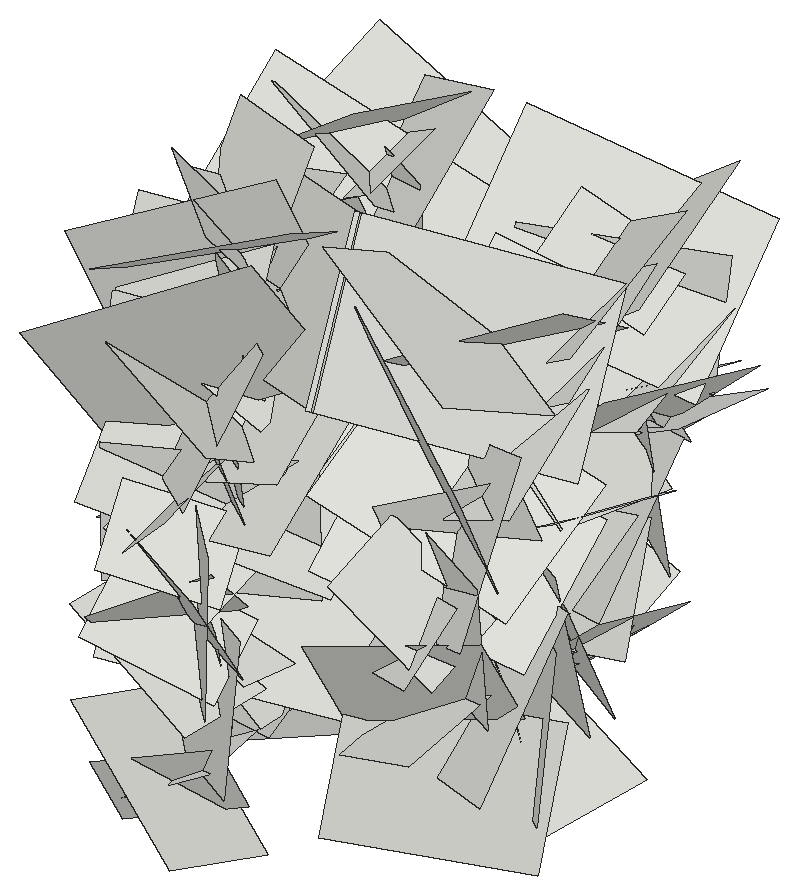
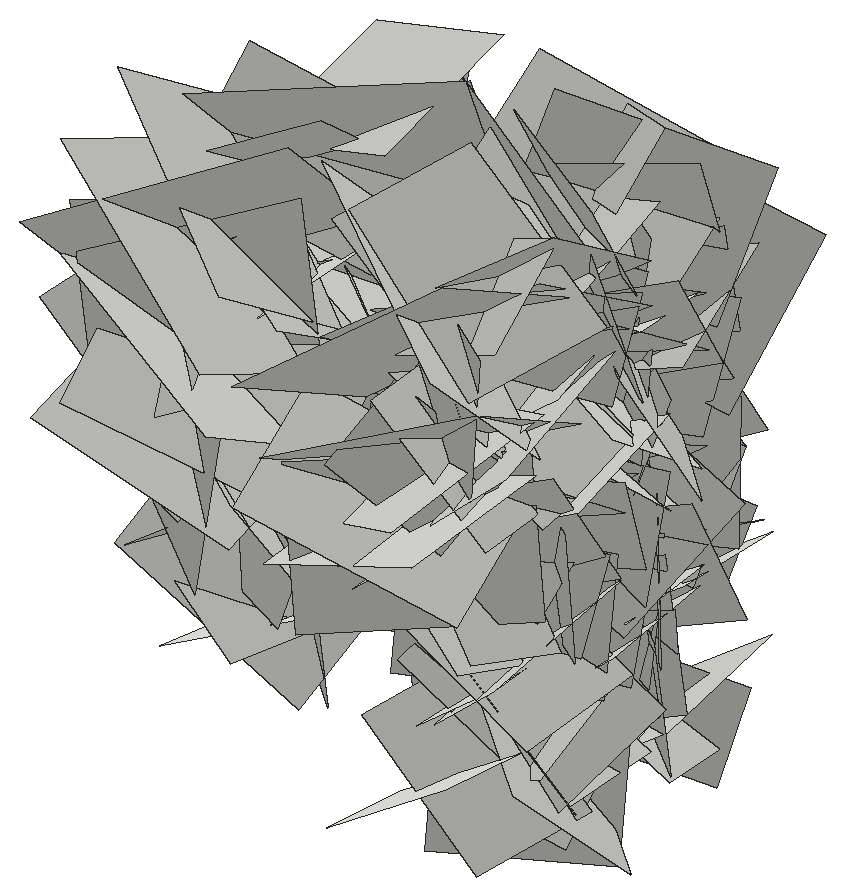
# SketchUp Ruby script. Lengths in inches.
U = 1.inch
M = Sketchup.active_model
def pt(a) = Geom::Point3d.new(a.map { |v| v * U })
def face(e, loops, mat)
  f = e.add_face(loops[0].map { |a| pt(a) })
  loops[1..].each { |l| e.add_face(l.map { |a| pt(a) }).erase! }
  f.material = f.back_material = mat if mat
  f
end
# faces: each face lists its corners as indices into pts; further lists are holes
def faces(e, pts, list, mat = nil) = list.each { |f| face(e, (f[0].is_a?(Array) ? f : [f]).map { |l| l.map { |i| pts[i] } }, mat) }
# xy, xz, yz: faces in a plane at the given z, y or x. An outline is a flat list of corners, or four numbers for a rectangle; further outlines are holes
def ring(l) = l.size == 4 ? [[l[0], l[1]], [l[2], l[1]], [l[2], l[3]], [l[0], l[3]]] : l.each_slice(2).to_a
def flat(e, list, mat, &to3) = list.each { |f| face(e, (f[0].is_a?(Array) ? f : [f]).map { |l| ring(l).map { |u, v| to3.(u, v) } }, mat) }
def xy(e, z, list, mat = nil) = flat(e, list, mat) { |x, y| [x, y, z] }
def xz(e, y, list, mat = nil) = flat(e, list, mat) { |x, z| [x, y, z] }
def yz(e, x, list, mat = nil) = flat(e, list, mat) { |y, z| [x, y, z] }
def lines(e, pts, list) = list.each { |a, b| e.add_line(pt(pts[a]), pt(pts[b])) }
# prism: a flat outline (further loops are holes) pulled along v
def prism(e, loops, v, mat = nil)
  f = face(e, loops, mat); d = Geom::Vector3d.new(v.map { |x| x * U })
  f.pushpull(f.normal.samedirection?(d) ? d.length : -d.length)
end
def box(e, o, s, mat = nil) = prism(e, [[o, [o[0] + s[0], o[1], o[2]], [o[0] + s[0], o[1] + s[1], o[2]], [o[0], o[1] + s[1], o[2]]]], [0, 0, s[2]], mat)
def at(x, y, z, deg = 0) = Geom::Transformation.translation(pt([x, y, z])) * Geom::Transformation.rotation(ORIGIN, Z_AXIS, deg.degrees)
def axes(o, x, y, z) = Geom::Transformation.new([*x, 0, *y, 0, *z, 0, *pt(o).to_a, 1])
def part(name) = M.definitions.add(name)
# library, detail: a bought-in or finely detailed component or shape, given as its bounding box
def library(name, o, s) = part(name).tap { |d| box(d.entities, o, s) }
def detail(e, o, s) = box(e.add_group.entities, o, s)
def put(e, d, t, mat = nil) = e.add_instance(d, t).tap { |i| i.material = mat if mat }
def group(e, t, mat = nil) = e.add_group.tap { |g| g.transformation = t; g.material = mat if mat }.entities
root = M.entities
c1 = part("Component\#6")
p = [[0.01,0,0],[0,3.24,4.54],[4.32,3.24,4.54],[4.33,0,0]]
faces(c1.entities,p,[[0,1,2,3]])
put(root,c1,axes([414.68,184.92,37.05],[-0.01613,-0.13323,-0.78421],[-0.01491,-0.78419,0.1335],[-0.84304,0.01642,0.01265]))
put(root,c1,axes([414.68,184.52,38.07],[0.06477,0.36641,0.7198],[-0.11209,0.71927,-0.35717],[-0.84878,-0.06703,0.10209]))
put(root,c1,axes([414.68,187.74,23.43],[0.08523,-0.9506,0.05636],[0.09187,0.06363,0.94959],[-1.00521,-0.07479,0.09156]))
put(root,c1,axes([410.71,187.08,35.11],[-0.23629,-0.52338,-1.02054],[-0.13084,-1.02265,0.55142],[1.20867,-0.21302,-0.13982]))
put(root,c1,axes([414.68,188.23,41.22],[0.26749,1.02168,-0.17372],[-0.00845,-0.17688,-1.05183],[-1.0985,0.25014,-0.03421]))
put(root,c1,axes([410.71,185.86,28.71],[-0.06844,0.29244,0.76285],[0.17475,0.75415,-0.27515],[0.84819,-0.13178,0.11824]))
put(root,c1,axes([410.71,192.58,32.17],[0.11188,-0.86522,-0.03173],[-0.14554,-0.04829,0.85998],[0.90613,0.09907,0.14204]))
put(root,c1,axes([410.71,189.53,40.3125],[-0.07096,0.70634,-0.4758],[0.12627,-0.46481,-0.70678],[0.89387,0.12173,0.06207]))
put(root,c1,axes([410.71,180.54,27.52],[0.00647,0.86334,-0.00303],[-0.00368,-0.003,-0.86336],[0.91514,-0.00612,-0.00345]))
put(root,c1,axes([414.68,184.84,39.1],[-0.02023,-0.20369,-0.6632],[-0.11732,-0.65406,0.20407],[-0.72599,0.11137,-0.0145]))
put(root,c1,axes([414.68,187.61,26.86],[0.07932,-0.16974,-0.83453],[0.0041,-0.83766,0.17072],[-0.9027,-0.01872,-0.07255]))
put(root,c1,axes([414.68,187.84,31.26],[-0.01205,0.8882,0.30464],[0.22592,0.29915,-0.86424],[-0.96935,0.05868,-0.20521]))
put(root,c1,axes([410.71,187.32,34.27],[0.05201,-0.4187,0.7383],[-0.02779,0.73844,0.42051],[0.89926,0.04704,-0.0297]))
put(root,c1,axes([414.68,182.78,23.92],[0.06221,-0.24398,0.83625],[0.07047,0.83695,0.23952],[-0.92069,0.04758,0.07484]))
put(root,c1,axes([410.71,186.99,20.26],[0.04681,-0.17583,0.86867],[-0.05724,0.86759,0.17835],[0.93771,0.06173,-0.03248]))
put(root,c1,axes([414.68,186.98,23.44],[0.07046,0.41434,0.63319],[-0.10971,0.63463,-0.40442],[-0.79457,-0.05088,0.11199]))
put(root,c1,axes([410.71,189.58,22.99],[-0.08755,-0.94666,0.34405],[-0.04779,0.34833,0.94763],[1.06661,-0.0621,0.0707]))
put(root,c1,axes([414.68,194.3125,23.26],[0.02367,-0.75059,-0.08188],[-0.02978,-0.08269,0.75031],[-0.79979,-0.01914,-0.03036]))
put(root,c1,axes([410.71,191.48,24.4],[-0.24044,-0.84726,-0.84182],[-0.11443,-0.83882,0.87332],[1.26085,-0.2377,-0.08127]))
put(root,c1,axes([410.71,182.91,34.72],[-0.14912,-0.41506,0.98502],[-0.044,0.99488,0.41329],[1.13217,-0.016,0.1458]))
put(root,c1,axes([414.68,183.3,35.54],[-0.06853,-0.0517,0.64839],[-0.02911,0.65122,0.04919],[-0.68886,-0.02238,-0.06659]))
put(root,c1,axes([414.68,186.9,33.68],[0.12726,-0.80704,-0.07778],[-0.05104,-0.08559,0.81372],[-0.85791,-0.11462,-0.05995]))
put(root,c1,axes([410.71,189.24,21.76],[0.15995,-0.688,0.38857],[-0.02017,0.39231,0.70202],[0.83731,0.14088,-0.05731]))
put(root,c1,axes([410.71,190.89,25.45],[-0.07637,-0.93381,0.1535],[0.06656,0.14888,0.93522],[1.00091,-0.08115,-0.05048]))
put(root,c1,axes([414.68,181.75,22.9],[-0.07496,0.59984,0.04506],[-0.05269,0.03939,-0.60235],[-0.63545,-0.07402,0.04463]))
put(root,c1,axes([410.71,186.8,27.07],[-0.11611,-1.02809,0.5245],[-0.14127,0.5346,1.02006],[1.21522,-0.03608,0.16869]))
put(root,c1,axes([414.68,189.49,31],[0.19159,0.03614,-0.77666],[-0.1449,-0.78347,-0.06827],[-0.81131,0.14846,-0.17121]))
put(root,c1,axes([414.68,188.48,31.6],[-0.00806,0.51701,-0.38199],[-0.06142,-0.38101,-0.51453],[-0.67861,0.02834,0.0511]))
put(root,c1,axes([410.71,182.86,27.86],[0.00866,0.87216,-0.09866],[0.12421,-0.09886,-0.86427],[0.92206,0.00513,0.11735]))
put(root,c1,axes([414.68,188.3,31.13],[0.1103,-0.11339,-0.88165],[0.13763,-0.87621,0.12802],[-0.93214,-0.14279,-0.08543]))
put(root,c1,axes([410.71,182.62,33.52],[-0.16113,0.63843,0.91206],[-0.00988,0.91976,-0.64538],[1.18006,0.09488,0.11913]))
put(root,c1,axes([410.71,186.85,26],[0.04759,0.74401,-0.43208],[0.09551,-0.43435,-0.73856],[0.90698,0.0067,0.10045]))
put(root,c1,axes([414.68,188.01,25.87],[0.18323,0.88768,-0.1275],[0.06793,-0.14175,-0.89995],[-0.94816,0.16139,-0.08912]))
put(root,c1,axes([414.68,181.88,29.24],[-0.0732,0.47057,-0.46808],[0.06498,-0.46407,-0.47558],[-0.70054,-0.09222,0.00479]))
put(root,c1,axes([414.68,186.27,36.66],[0.23271,0.08267,-1.0169],[0.17131,-1.02986,-0.04883],[-1.06781,-0.14721,-0.22945]))
put(root,c1,axes([414.68,182.11,23.57],[0.01533,0.32032,-0.55846],[-0.07998,-0.55391,-0.31966],[-0.67773,0.07262,0.02509]))
put(root,c1,axes([410.71,181.12,36.49],[-0.0887,0.85058,-0.45713],[0.14057,-0.44437,-0.85112],[1.01388,0.13603,0.07801]))
put(root,c1,axes([410.71,184.8,33.37],[0.19651,0.19461,-0.78555],[-0.01158,-0.80522,-0.20206],[0.85778,-0.05545,0.17724]))
put(root,c1,axes([410.71,180.55,24.45],[0.04702,0.95483,-0.28451],[-0.08229,-0.28062,-0.95386],[1.05288,-0.06457,-0.06184]))
put(root,c1,axes([410.71,186.48,30.64],[0.03295,0.70699,0.47041],[0.18441,0.45544,-0.69599],[0.88105,-0.12176,0.12808]))
put(root,c1,axes([414.68,184.65,28.76],[-0.04824,-0.62434,-0.28052],[0.09786,-0.28417,0.61748],[-0.7189,0.00321,0.10288]))
put(root,c1,axes([414.68,188.62,32.29],[0.0866,-0.74743,0.19758],[0.06186,0.20408,0.74787],[-0.81715,-0.06376,0.07755]))
put(root,c1,axes([414.68,183.74,37.84],[-0.08456,-0.37494,0.46177],[0.03825,0.46199,0.38136],[-0.62935,0.07846,-0.03886]))
put(root,c1,axes([410.71,185.4,30.76],[-0.02152,-0.00963,-1.2106],[-0.23963,-1.18945,0.01326],[1.26071,-0.22625,-0.01814]))
put(root,c1,axes([410.71,187.18,35.87],[-0.21905,1.32848,-0.23139],[-0.18572,-0.25856,-1.32798],[1.41727,0.17144,-0.20979]))
put(root,c1,axes([414.68,188.41,35.3125],[-0.03073,0.48255,0.4704],[0.10717,0.46862,-0.47449],[-0.70624,0.05011,-0.09248]))
put(root,c1,axes([414.68,183.98,26.9],[0.15473,-0.64925,-0.29626],[-0.07231,-0.3137,0.65387],[-0.75301,-0.10329,-0.12366]))
put(root,c1,axes([414.68,183.4375,30.23],[0.10865,-0.24445,0.66529],[-0.00738,0.67183,0.24793],[-0.75127,-0.04195,0.09378]))
put(root,c1,axes([414.68,185.35,37.93],[0.06077,0.5182,0.40006],[-0.00909,0.40215,-0.51968],[-0.69387,0.04012,0.04185]))
put(root,c1,axes([410.71,182.41,31.86],[-0.21699,-0.67676,1.03332],[0.0082,1.04669,0.68705],[1.3093,-0.11872,0.16695]))
put(root,c1,axes([410.71,181.64,30.57],[0.02444,0.48831,-0.77146],[0.19424,-0.75848,-0.47462],[0.9481,0.1428,0.11713]))
put(root,c1,axes([410.71,184.85,32.98],[-0.15473,1.07562,-0.16592],[0.16403,-0.14519,-1.07739],[1.14193,0.1666,0.13228]))
put(root,c1,axes([414.68,179.78,31.84],[0.01485,0.68647,0.23212],[0.1576,0.2245,-0.67291],[-0.75179,0.06062,-0.13648]))
put(root,c1,axes([414.68,188.93,38.32],[0.06934,0.59373,0.25],[-0.00198,0.25145,-0.59671],[-0.68287,0.05956,0.02711]))
put(root,c1,axes([414.68,193.29,29.97],[-0.02765,-0.60791,0.13872],[0.08921,0.13414,0.60366],[-0.6549,0.04394,0.07638]))
put(root,c1,axes([410.71,189.07,22.99],[0.09993,-0.91741,-0.05408],[0.10319,-0.04408,0.91762],[0.96866,0.09934,-0.09218]))
put(root,c1,axes([410.71,185.63,37.94],[-0.10296,1.07287,0.66666],[-0.13207,0.65722,-1.07584],[1.33238,0.14805,-0.05512]))
put(root,c1,axes([410.71,185.55,26.35],[0.05433,-0.24183,-1.04679],[-0.06418,-1.04696,0.23891],[1.13701,-0.04754,0.0635]))
put(root,c1,axes([414.68,186.02,29.02],[0.12909,0.32312,-0.64935],[0.06195,-0.66067,-0.31779],[-0.76632,0.00102,-0.13508]))
put(root,c1,axes([410.71,190.19,31.82],[0.07854,-1.04848,0.11995],[-0.05802,0.11627,1.05008],[1.11713,0.07975,0.0461]))
put(root,c1,axes([414.68,188.83,29.07],[0.04972,0.59189,0.16701],[0.02122,0.16593,-0.59371],[-0.65156,0.05057,-0.00659]))
put(root,c1,axes([410.71,185.29,39.56],[0.11827,0.82487,-0.51088],[0.03346,-0.51706,-0.82795],[1.02793,-0.07808,0.08573]))
put(root,c1,axes([410.71,186.92,28.87],[0.11772,1.08189,-0.3436],[-0.18933,-0.32428,-1.0788],[1.18826,-0.15885,-0.13785]))
put(root,c1,axes([414.68,191.45,35.51],[0.13227,0.51495,-0.41011],[0.00116,-0.41758,-0.52399],[-0.6978,0.09692,-0.07861]))
put(root,c1,axes([414.68,183.51,30.36],[0.10644,-0.42009,-0.4575],[-0.01901,-0.46521,0.42323],[-0.65811,-0.0545,-0.08622]))
put(root,c1,axes([410.71,184.16,23.6],[0.00632,0.19994,1.20323],[-0.15077,1.19515,-0.1979],[1.28409,0.13934,-0.02916]))
put(root,c1,axes([410.71,189.26,31.29],[0.07003,-0.18149,-1.00879],[0.05402,-1.00905,0.18487],[1.08514,0.06195,0.0559]))
put(root,c1,axes([414.68,191.07,24.72],[0.08022,-0.60182,-0.03468],[0.03515,-0.03074,0.60586],[-0.63802,-0.07736,0.02902]))
put(root,c1,axes([410.71,187.65,25.55],[0.14301,-0.32766,0.90945],[0.11586,0.91755,0.31436],[1.01811,-0.05839,-0.16352]))
put(root,c1,axes([410.71,192.86,38.11],[0.10772,-0.0541,-1.0459],[0.04447,-1.04976,0.05837],[1.10925,0.04734,0.09923]))
put(root,c1,axes([414.68,188.74,27.6],[0.13014,-0.45431,-0.37588],[0.00674,-0.3829,0.46487],[-0.62498,-0.09873,-0.07326]))
put(root,c1,axes([410.71,181.98,27.65],[0.03848,-0.07343,1.06513],[0.13392,1.05855,0.06867],[1.12376,-0.12364,-0.04466]))
put(root,c1,axes([410.71,182.88,33.98],[0.05541,0.90127,0.55592],[0.17138,0.54328,-0.89597],[1.1093,-0.12895,0.11065]))
put(root,c1,axes([410.71,190.1,29],[0.15352,-0.05709,1.12322],[-0.06907,1.13017,0.06585],[1.19015,0.07295,-0.14107]))
put(root,c1,axes([410.71,185.59,36.56],[0.07365,1.00309,0.56692],[0.00038,0.56794,-1.00493],[1.22135,-0.06067,-0.03387]))
put(root,c1,axes([410.71,194.96,38.36],[-0.08597,-0.96025,-0.92678],[-0.03419,-0.92681,0.9631],[1.41421,-0.08078,-0.03305]))
put(root,c1,axes([410.71,188.57,34.3],[-0.02784,1.05016,0.5271],[0.1514,0.52617,-1.0412],[1.23628,-0.04079,0.13938]))
put(root,c1,axes([410.71,186.91,28.91],[-0.08475,0.77289,1.06783],[0.0494,1.07079,-0.77154],[1.39641,0.00903,0.0921]))
put(root,c1,axes([410.71,187.29,32.09],[-0.03087,-0.89426,-0.74249],[0.26998,-0.72958,0.86873],[1.20212,0.14089,-0.21417]))
put(root,c1,axes([410.71,190.5,33.59],[0.11278,1.05886,-0.21225],[0.21462,-0.22906,-1.04119],[1.12442,-0.06248,0.22002]))
put(root,c1,axes([410.71,184.99,36.41],[0.13687,-0.99381,0.45239],[0.15227,0.46704,0.985],[1.14738,0.05657,-0.18469]))
put(root,c1,axes([410.71,181.61,25.33],[-0.14764,0.72138,1.18272],[0.09804,1.19088,-0.71546],[1.46521,-0.007,0.16705]))
put(root,c1,axes([410.71,187.26,33.24],[0.066,-0.95024,-0.64083],[0.19237,-0.6255,0.94515],[1.19957,0.15259,-0.11631]))
put(root,c1,axes([410.71,188.72,38.18],[0.108,1.17484,0.54266],[-0.09899,0.5496,-1.17232],[1.36819,-0.05298,-0.12766]))
put(root,c1,axes([410.71,180.73,30.67],[0.05707,0.69485,1.12415],[-0.04583,1.1254,-0.69356],[1.4001,0.00851,-0.06852]))
put(root,c1,axes([410.71,193.84,30.46],[0.25587,-1.06575,0.3461],[0.15582,0.3811,1.07099],[1.17751,0.18115,-0.21693]))
put(root,c1,axes([410.71,188.1875,39.24],[0.00053,-0.50504,-1.25708],[0.1621,-1.24903,0.50186],[1.42684,0.14209,-0.05655]))
put(root,c1,axes([410.71,186.51,25.44],[-0.00901,-0.3677,1.34811],[0.26845,1.32541,0.3631],[1.45667,-0.24653,-0.05858]))
put(root,c1,axes([410.71,190.14,35.27],[0.30668,1.10496,-0.445],[0.14325,-0.48543,-1.11748],[1.25452,-0.21469,0.23639]))
put(root,c1,axes([424.49,190.14,35.27],[-0.30668,1.10496,-0.445],[-0.14325,-0.48543,-1.11748],[-1.25452,-0.21469,0.23639]))
put(root,c1,axes([424.49,186.51,25.44],[0.00901,-0.3677,1.34811],[-0.26845,1.32541,0.3631],[-1.45667,-0.24653,-0.05858]))
put(root,c1,axes([424.49,188.1875,39.24],[-0.00053,-0.50504,-1.25708],[-0.1621,-1.24903,0.50186],[-1.42684,0.14209,-0.05655]))
put(root,c1,axes([424.49,180.73,30.67],[-0.05707,0.69485,1.12415],[0.04583,1.1254,-0.69356],[-1.4001,0.00851,-0.06852]))
put(root,c1,axes([424.49,188.72,38.18],[-0.108,1.17484,0.54266],[0.09899,0.5496,-1.17232],[-1.36819,-0.05298,-0.12766]))
put(root,c1,axes([424.49,187.26,33.24],[-0.066,-0.95024,-0.64083],[-0.19237,-0.6255,0.94515],[-1.19957,0.15259,-0.11631]))
put(root,c1,axes([424.49,181.61,25.33],[0.14764,0.72138,1.18272],[-0.09804,1.19088,-0.71546],[-1.46521,-0.007,0.16705]))
put(root,c1,axes([424.49,184.99,36.41],[-0.13687,-0.99381,0.45239],[-0.15227,0.46704,0.985],[-1.14738,0.05657,-0.18469]))
put(root,c1,axes([424.49,190.5,33.59],[-0.11278,1.05886,-0.21225],[-0.21462,-0.22906,-1.04119],[-1.12442,-0.06248,0.22002]))
put(root,c1,axes([424.49,187.29,32.09],[0.03087,-0.89426,-0.74249],[-0.26998,-0.72958,0.86873],[-1.20212,0.14089,-0.21417]))
put(root,c1,axes([424.49,186.91,28.91],[0.08475,0.77289,1.06783],[-0.0494,1.07079,-0.77154],[-1.39641,0.00903,0.0921]))
put(root,c1,axes([424.49,188.57,34.3],[0.02784,1.05016,0.5271],[-0.1514,0.52617,-1.0412],[-1.23628,-0.04079,0.13938]))
put(root,c1,axes([424.49,194.96,38.36],[0.08597,-0.96025,-0.92678],[0.03419,-0.92681,0.9631],[-1.41421,-0.08078,-0.03305]))
put(root,c1,axes([424.49,185.59,36.56],[-0.07365,1.00309,0.56692],[-0.00038,0.56794,-1.00493],[-1.22135,-0.06067,-0.03387]))
put(root,c1,axes([424.49,190.1,29],[-0.15352,-0.05709,1.12322],[0.06907,1.13017,0.06585],[-1.19015,0.07295,-0.14107]))
put(root,c1,axes([424.49,182.88,33.98],[-0.05541,0.90127,0.55592],[-0.17138,0.54328,-0.89597],[-1.1093,-0.12895,0.11065]))
put(root,c1,axes([424.49,181.98,27.65],[-0.03848,-0.07343,1.06513],[-0.13392,1.05855,0.06867],[-1.12376,-0.12364,-0.04466]))
put(root,c1,axes([420.52,188.74,27.6],[-0.13014,-0.45431,-0.37588],[-0.00674,-0.3829,0.46487],[0.62498,-0.09873,-0.07326]))
put(root,c1,axes([424.49,192.86,38.11],[-0.10772,-0.0541,-1.0459],[-0.04447,-1.04976,0.05837],[-1.10925,0.04734,0.09923]))
put(root,c1,axes([424.49,187.65,25.55],[-0.14301,-0.32766,0.90945],[-0.11586,0.91755,0.31436],[-1.01811,-0.05839,-0.16352]))
put(root,c1,axes([420.52,191.07,24.72],[-0.08022,-0.60182,-0.03468],[-0.03515,-0.03074,0.60586],[0.63802,-0.07736,0.02902]))
put(root,c1,axes([424.49,189.26,31.29],[-0.07003,-0.18149,-1.00879],[-0.05402,-1.00905,0.18487],[-1.08514,0.06195,0.0559]))
put(root,c1,axes([424.49,184.16,23.6],[-0.00632,0.19994,1.20323],[0.15077,1.19515,-0.1979],[-1.28409,0.13934,-0.02916]))
put(root,c1,axes([420.52,183.51,30.36],[-0.10644,-0.42009,-0.4575],[0.01901,-0.46521,0.42323],[0.65811,-0.0545,-0.08622]))
put(root,c1,axes([420.52,191.45,35.51],[-0.13227,0.51495,-0.41011],[-0.00116,-0.41758,-0.52399],[0.6978,0.09692,-0.07861]))
put(root,c1,axes([424.49,186.92,28.87],[-0.11772,1.08189,-0.3436],[0.18933,-0.32428,-1.0788],[-1.18826,-0.15885,-0.13785]))
put(root,c1,axes([424.49,185.29,39.56],[-0.11827,0.82487,-0.51088],[-0.03346,-0.51706,-0.82795],[-1.02793,-0.07808,0.08573]))
put(root,c1,axes([420.52,188.83,29.07],[-0.04972,0.59189,0.16701],[-0.02122,0.16593,-0.59371],[0.65156,0.05057,-0.00659]))
put(root,c1,axes([424.49,190.19,31.82],[-0.07854,-1.04848,0.11995],[0.05802,0.11627,1.05008],[-1.11713,0.07975,0.0461]))
put(root,c1,axes([420.52,186.02,29.02],[-0.12909,0.32312,-0.64935],[-0.06195,-0.66067,-0.31779],[0.76632,0.00102,-0.13508]))
put(root,c1,axes([424.49,185.55,26.35],[-0.05433,-0.24183,-1.04679],[0.06418,-1.04696,0.23891],[-1.13701,-0.04754,0.0635]))
put(root,c1,axes([424.49,185.63,37.94],[0.10296,1.07287,0.66666],[0.13207,0.65722,-1.07584],[-1.33238,0.14805,-0.05512]))
put(root,c1,axes([424.49,189.07,22.99],[-0.09993,-0.91741,-0.05408],[-0.10319,-0.04408,0.91762],[-0.96866,0.09934,-0.09218]))
put(root,c1,axes([420.52,193.29,29.97],[0.02765,-0.60791,0.13872],[-0.08921,0.13414,0.60366],[0.6549,0.04394,0.07638]))
put(root,c1,axes([420.52,188.93,38.32],[-0.06934,0.59373,0.25],[0.00198,0.25145,-0.59671],[0.68287,0.05956,0.02711]))
put(root,c1,axes([420.52,179.78,31.84],[-0.01485,0.68647,0.23212],[-0.1576,0.2245,-0.67291],[0.75179,0.06062,-0.13648]))
put(root,c1,axes([424.49,184.85,32.98],[0.15473,1.07562,-0.16592],[-0.16403,-0.14519,-1.07739],[-1.14193,0.1666,0.13228]))
put(root,c1,axes([424.49,181.64,30.57],[-0.02444,0.48831,-0.77146],[-0.19424,-0.75848,-0.47462],[-0.9481,0.1428,0.11713]))
put(root,c1,axes([424.49,182.41,31.86],[0.21699,-0.67676,1.03332],[-0.0082,1.04669,0.68705],[-1.3093,-0.11872,0.16695]))
put(root,c1,axes([420.52,185.35,37.93],[-0.06077,0.5182,0.40006],[0.00909,0.40215,-0.51968],[0.69387,0.04012,0.04185]))
put(root,c1,axes([420.52,183.4375,30.23],[-0.10865,-0.24445,0.66529],[0.00738,0.67183,0.24793],[0.75127,-0.04195,0.09378]))
put(root,c1,axes([420.52,183.98,26.9],[-0.15473,-0.64925,-0.29626],[0.07231,-0.3137,0.65387],[0.75301,-0.10329,-0.12366]))
put(root,c1,axes([420.52,188.41,35.3125],[0.03073,0.48255,0.4704],[-0.10717,0.46862,-0.47449],[0.70624,0.05011,-0.09248]))
put(root,c1,axes([424.49,187.18,35.87],[0.21905,1.32848,-0.23139],[0.18572,-0.25856,-1.32798],[-1.41727,0.17144,-0.20979]))
